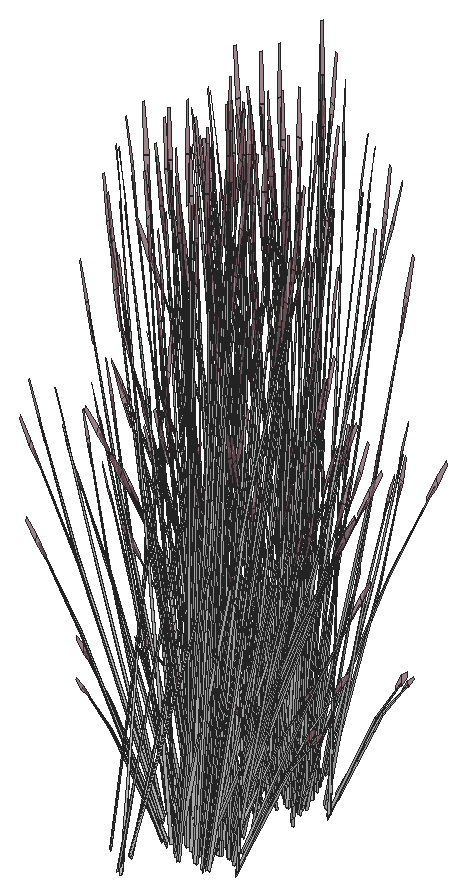
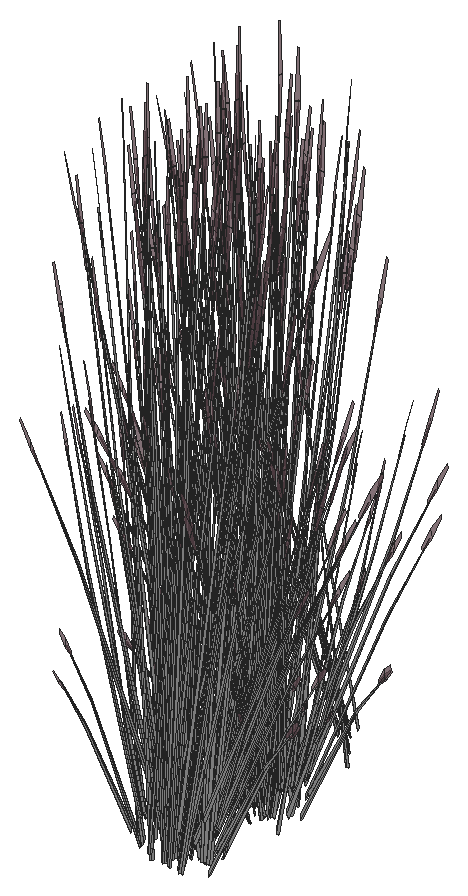
# SketchUp Ruby script. Lengths in inches.
U = 1.inch
M = Sketchup.active_model
def pt(a) = Geom::Point3d.new(a.map { |v| v * U })
def face(e, loops, mat)
  f = e.add_face(loops[0].map { |a| pt(a) })
  loops[1..].each { |l| e.add_face(l.map { |a| pt(a) }).erase! }
  f.material = f.back_material = mat if mat
  f
end
# faces: each face lists its corners as indices into pts; further lists are holes
def faces(e, pts, list, mat = nil) = list.each { |f| face(e, (f[0].is_a?(Array) ? f : [f]).map { |l| l.map { |i| pts[i] } }, mat) }
# xy, xz, yz: faces in a plane at the given z, y or x. An outline is a flat list of corners, or four numbers for a rectangle; further outlines are holes
def ring(l) = l.size == 4 ? [[l[0], l[1]], [l[2], l[1]], [l[2], l[3]], [l[0], l[3]]] : l.each_slice(2).to_a
def flat(e, list, mat, &to3) = list.each { |f| face(e, (f[0].is_a?(Array) ? f : [f]).map { |l| ring(l).map { |u, v| to3.(u, v) } }, mat) }
def xy(e, z, list, mat = nil) = flat(e, list, mat) { |x, y| [x, y, z] }
def xz(e, y, list, mat = nil) = flat(e, list, mat) { |x, z| [x, y, z] }
def yz(e, x, list, mat = nil) = flat(e, list, mat) { |y, z| [x, y, z] }
def lines(e, pts, list) = list.each { |a, b| e.add_line(pt(pts[a]), pt(pts[b])) }
# prism: a flat outline (further loops are holes) pulled along v
def prism(e, loops, v, mat = nil)
  f = face(e, loops, mat); d = Geom::Vector3d.new(v.map { |x| x * U })
  f.pushpull(f.normal.samedirection?(d) ? d.length : -d.length)
end
def box(e, o, s, mat = nil) = prism(e, [[o, [o[0] + s[0], o[1], o[2]], [o[0] + s[0], o[1] + s[1], o[2]], [o[0], o[1] + s[1], o[2]]]], [0, 0, s[2]], mat)
def at(x, y, z, deg = 0) = Geom::Transformation.translation(pt([x, y, z])) * Geom::Transformation.rotation(ORIGIN, Z_AXIS, deg.degrees)
def axes(o, x, y, z) = Geom::Transformation.new([*x, 0, *y, 0, *z, 0, *pt(o).to_a, 1])
def part(name) = M.definitions.add(name)
# library, detail: a bought-in or finely detailed component or shape, given as its bounding box
def library(name, o, s) = part(name).tap { |d| box(d.entities, o, s) }
def detail(e, o, s) = box(e.add_group.entities, o, s)
def put(e, d, t, mat = nil) = e.add_instance(d, t).tap { |i| i.material = mat if mat }
def group(e, t, mat = nil) = e.add_group.tap { |g| g.transformation = t; g.material = mat if mat }.entities
root = M.entities
M.materials.add("LightPink_Translucent").color = [144, 107, 117]
M.materials["LightPink_Translucent"].alpha = 0.75
M.materials.add("[_0053_Ivory_]").color = [200, 200, 200]
c1 = part("blade")
p = [[2.15,0.21,22],[0,0.17,0],[0.09,0.45,0],[2.18,0.31,22],[2.29,0.31,22],[0.38,0.45,0],
  [2.48,0.24,33],[2.49,0.24,33],[2.48,0.22,33]]
faces(c1.entities,p,[[0,1,2,3],[4,5,2,3],[6,3,4,7],[8,0,3,6]])
c2 = part("seeds")
p = [[0.3,-0.1,1.38],[-0.01,-0.03,1.59],[-0.01,-0.03,0.03],[0.14,-0.07,-0.07],[0.29,-0.03,3],[0.15,0.01,3.11]]
faces(c2.entities,p,[[0,1,2,3],[1,0,4,5]],"LightPink_Translucent")
c3 = part("blade with seeds")
put(c3.entities,c1,at(0,0,0))
put(c3.entities,c2,axes([2.4,0.25,30.99],[1.5799,-0.05474,1.17369],[-0.12525,1.92788,0.29478],[-0.07173,-0.02425,1.56792]))
put(root,c3,axes([679.4,325.39,38.18],[-0.1831,0.48359,-0.35414],[-0.53419,-0.14105,0.4572],[0.04898,0.1947,0.87481]),"[_0053_Ivory_]")
put(root,c3,axes([677.35,331.33,36.24],[0.11858,0.17508,1.43002],[-0.27325,0.4759,-0.30754],[-0.28057,-0.11375,0.61141]),"[_0053_Ivory_]")
put(root,c3,axes([679.41,330.5,35.68],[0.56663,0.1556,-0.30978],[-0.14267,0.54795,0.30978],[0.11423,-0.06319,1.38974]),"[_0053_Ivory_]")
put(root,c3,axes([678.25,324.45,38.99],[-0.0158,0.58168,-0.7886],[-0.66548,-0.03907,0.09517],[-0.07023,0.24643,1.11556]),"[_0053_Ivory_]")
put(root,c3,axes([677.83,331.17,38.63],[-0.60713,-0.01514,-0.71045],[0.04078,-0.63759,0.08574],[-0.25721,-0.06729,1.00501]),"[_0053_Ivory_]")
put(root,c3,axes([678.88,324.04,37.53],[-0.01487,-0.24136,1.71376],[0.64429,0.16012,0.13857],[-0.03985,0.34396,0.73262]),"[_0053_Ivory_]")
put(root,c3,axes([679.46,324.95,38.63],[0.28988,0.51132,-0.71045],[-0.59671,0.28496,0.08574],[0.06778,0.24706,1.00501]),"[_0053_Ivory_]")
put(root,c3,axes([677.8,332.4,35.98],[-0.56493,0.5287,0.30756],[-0.56528,-0.52313,-0.36492],[-0.01973,-0.15014,1.64885]),"[_0053_Ivory_]")
put(root,c3,axes([677.78,325.76,36.24],[0.19166,-0.0992,1.43002],[0.4732,0.29912,-0.30754],[-0.14084,0.25882,0.61141]),"[_0053_Ivory_]")
put(root,c3,axes([679.6,332.65,36.09],[0.68433,0.30479,0.24065],[-0.32934,0.63331,0.50002],[0,-0.14599,1.60543]),"[_0053_Ivory_]")
put(root,c3,axes([679.33,333.5,36.09],[0.16098,-0.74515,-0.23429],[0.76326,0.12989,0.51271],[-0.13337,-0.1029,1.5644]),"[_0053_Ivory_]")
put(root,c3,axes([677.63,331.3,38.33],[-0.44101,0.41656,-0.51099],[-0.38623,-0.44004,-0.3958],[-0.22407,-0.06338,0.97773]),"[_0053_Ivory_]")
put(root,c3,axes([676.64,331.86,36.42],[0.38775,-0.045,1.1486],[-0.24596,0.39648,0.84392],[-0.19161,-0.05948,0.25299]),"[_0053_Ivory_]")
put(root,c3,axes([679.38,332.22,36.37],[-0.65953,0.03882,0.44739],[-0.05964,-0.64439,-0.21531],[0.11807,-0.06531,1.43643]),"[_0053_Ivory_]")
put(root,c3,axes([677.68,332.69,36.13],[0,0.62885,0.49651],[-0.67951,0,0],[0,-0.14322,1.57504]),"[_0053_Ivory_]")
put(root,c3,axes([682.45,332.83,38.33],[0.16454,-0.57202,-0.51099],[0.56413,0.19607,-0.3958],[0.22713,-0.05245,0.97773]),"[_0053_Ivory_]")
put(root,c3,axes([678.03,325.27,37.02],[0.01334,-0.32463,1.54345],[0.60018,0.17147,0.21329],[-0.052,0.34598,0.72882]),"[_0053_Ivory_]")
put(root,c3,axes([681.55,330.5,36.03],[0.37973,-0.63014,0],[0.6353,0.35142,-0.51607],[0.14469,0.08004,1.63711]),"[_0053_Ivory_]")
put(root,c3,axes([677.08,331.75,37.53],[0.25192,-0.01424,1.71376],[-0.16712,0.61729,0.13857],[-0.35901,-0.03818,0.73262]),"[_0053_Ivory_]")
put(root,c3,axes([679.28,333.2,35.86],[-0.36485,-0.52782,-0.44739],[0.55265,-0.37168,0.21531],[-0.11807,-0.06531,1.43643]),"[_0053_Ivory_]")
put(root,c3,axes([679.36,332.45,36.01],[0.26406,0.70318,0.45755],[-0.7545,0.24452,0.17955],[0.00922,-0.12921,1.58856]),"[_0053_Ivory_]")
put(root,c3,axes([683.05,332.99,35.64],[-0.39118,0.07547,1.41583],[-0.06226,-0.6007,0.08104],[0.27398,-0.09092,0.80566]),"[_0053_Ivory_]")
put(root,c3,axes([683.76,332.46,35.91],[-0.37654,-0.40212,-0.06488],[0.4124,-0.36845,-0.29416],[0.11685,-0.02594,0.97024]),"[_0053_Ivory_]")
put(root,c3,axes([679.22,333.01,36.37],[-0.29468,0.56664,0.44739],[-0.61229,-0.27271,-0.21531],[0,-0.13062,1.43643]),"[_0053_Ivory_]")
put(root,c3,axes([680.31,332.51,35.86],[0,-0.72763,0],[0.75945,0,0],[0,0,1.79456]),"[_0053_Ivory_]")
put(root,c3,axes([681.23,330.83,36.13],[-0.56842,-0.31443,0.49651],[0.33976,-0.56381,0],[0.12946,0.07161,1.57504]),"[_0053_Ivory_]")
put(root,c3,axes([682.34,333.04,38.63],[0.53369,-0.27773,-0.71045],[0.29743,0.5717,0.08574],[0.25786,-0.06494,1.00501]),"[_0053_Ivory_]")
put(root,c3,axes([678.95,333.4,35.71],[-0.63179,-0.1031,-0.62353],[0.13332,-0.63596,-0.16365],[-0.18854,-0.07706,1.37633]),"[_0053_Ivory_]")
put(root,c3,axes([679.95,332.06,36.01],[-0.50358,0.57069,0.45755],[-0.59827,-0.50377,0.17955],[0.1214,-0.05695,1.58856]),"[_0053_Ivory_]")
put(root,c3,axes([680.5,333.08,35.95],[-0.56493,-0.54126,-0.06131],[0.56528,-0.54159,0],[-0.01973,-0.0189,1.75571]),"[_0053_Ivory_]")
put(root,c3,axes([679.07,331.12,36.13],[-0.17545,0.62497,0.17642],[-0.64204,-0.17686,0.35086],[0.11091,-0.00304,1.60407]),"[_0053_Ivory_]")
put(root,c3,axes([678.81,331.62,35.25],[-0.59782,0.25177,1.28929],[-0.19028,-0.72239,0.50096],[0.36709,0.01202,1.46642]),"[_0053_Ivory_]")
put(root,c3,axes([680.41,331.8125,36.27],[0.11717,-0.56122,0.1448],[0.57245,0.09742,-0.41347],[0.10418,0.05763,1.26744]),"[_0053_Ivory_]")
put(root,c3,axes([679.42,333.14,36.01],[0.76764,0.13249,0.45755],[-0.15622,0.74829,0.17955],[-0.11218,-0.07226,1.58856]),"[_0053_Ivory_]")
put(root,c3,axes([683.48,332.6,35.15],[-0.03174,-0.09547,1.76342],[0.22015,-0.55846,-0.26939],[0.22208,-0.00803,0.30037]),"[_0053_Ivory_]")
put(root,c3,axes([676.92,332.5,35.15],[0.0154,0.09911,1.76342],[-0.31051,0.51756,-0.26939],[-0.22056,-0.02609,0.30037]),"[_0053_Ivory_]")
put(root,c3,axes([680.17,331.96,36.37],[-0.36485,-0.52782,0.44739],[0.55265,-0.37168,-0.21531],[0.11807,0.06531,1.43643]),"[_0053_Ivory_]")
put(root,c3,axes([678.28,334.37,35.68],[-0.14267,-0.54795,-0.30978],[0.56663,-0.1556,0.30978],[-0.11423,-0.06319,1.38974]),"[_0053_Ivory_]")
put(root,c3,axes([679.01,334.34,36.13],[0.65264,-0.16691,0.17642],[0.16115,0.62115,0.35086],[-0.05821,-0.0905,1.60407]),"[_0053_Ivory_]")
put(root,c3,axes([680.35,331.99,36.32],[0.61322,-0.4175,-0.29095],[0.40778,0.58992,-0.50002],[0.1513,0.05991,1.59708]),"[_0053_Ivory_]")
put(root,c3,axes([682.79,333.09,38.18],[0.50475,0.17543,-0.35414],[-0.14722,0.5118,0.4572],[0.20322,-0.04693,0.87481]),"[_0053_Ivory_]")
put(root,c3,axes([678.125,334.61,35.67],[-0.56842,-0.31443,-0.49651],[0.33976,-0.56381,0],[-0.12946,-0.07161,1.57504]),"[_0053_Ivory_]")
put(root,c3,axes([681.9,330.88,35.67],[0.56842,0.31443,-0.49651],[-0.33976,0.56381,0],[0.12946,0.07161,1.57504]),"[_0053_Ivory_]")
put(root,c3,axes([676.86,332.28,38.18],[-0.50475,-0.17543,-0.35414],[0.14722,-0.5118,0.4572],[-0.20322,0.04693,0.87481]),"[_0053_Ivory_]")
put(root,c3,axes([680.82,332.68,35.86],[0.67951,0,0],[0,0.65103,0],[0,0,1.78407]),"[_0053_Ivory_]")
put(root,c3,axes([679.67,333.5,36.32],[-0.61322,0.4175,-0.29095],[-0.40778,-0.58992,-0.50002],[-0.1513,-0.05991,1.59708]),"[_0053_Ivory_]")
put(root,c3,axes([681.01,331.15,36.13],[-0.65264,0.16691,0.17642],[-0.16115,-0.62115,0.35086],[0.05821,0.0905,1.60407]),"[_0053_Ivory_]")
put(root,c3,axes([681.42,332.46,37.53],[-0.25192,0.01424,1.71376],[0.16712,-0.61729,0.13857],[0.35901,0.03818,0.73262]),"[_0053_Ivory_]")
put(root,c3,axes([681.74,331.12,35.68],[0.14267,0.54795,-0.30978],[-0.56663,0.1556,0.30978],[0.11423,0.06319,1.38974]),"[_0053_Ivory_]")
put(root,c3,axes([680.6,332.35,36.03],[-0.76764,-0.13249,0.49198],[0.15622,-0.74829,0.19306],[0.11218,0.07226,1.70813]),"[_0053_Ivory_]")
put(root,c3,axes([679.99,334.19,35.86],[-0.19817,-0.54216,0],[0.56587,-0.18986,0],[0,0,1.54371]),"[_0053_Ivory_]")
put(root,c3,axes([679.61,333.68,36.27],[-0.11717,0.56122,0.1448],[-0.57245,-0.09742,-0.41347],[-0.10418,-0.05763,1.26744]),"[_0053_Ivory_]")
put(root,c3,axes([680.73,334.12,35.84],[0.63764,-0.21337,-0.19198],[0.22406,0.61462,0.00008],[0.07038,-0.02358,1.73897]),"[_0053_Ivory_]")
put(root,c3,axes([680.95,334.375,36.13],[0.17545,-0.62497,0.17642],[0.64204,0.17686,0.35086],[-0.11091,0.00304,1.60407]),"[_0053_Ivory_]")
put(root,c3,axes([680.81,332.96,35.87],[0.42396,0.40619,0],[-0.42396,0.40619,0],[0,0,1.69266]),"[_0053_Ivory_]")
put(root,c3,axes([678.4,332.19,37],[0.17264,-0.09097,1.77064],[0.05953,0.63516,0.13857],[-0.37394,0.08428,0.63284]),"[_0053_Ivory_]")
put(root,c3,axes([681.95,332.78,36.13],[-0.47719,-0.45806,0.17642],[0.48088,-0.44429,0.35086],[-0.0527,0.09355,1.60407]),"[_0053_Ivory_]")
put(root,c3,axes([681.07,332.09,35.71],[0.63179,0.1031,-0.62353],[-0.13332,0.63596,-0.16365],[0.18854,0.07706,1.37633]),"[_0053_Ivory_]")
put(root,c3,axes([683.86,333.2,36.42],[-0.37526,0.10382,1.1486],[0.17664,-0.42906,0.84392],[0.19907,0.02936,0.25299]),"[_0053_Ivory_]")
put(root,c3,axes([679.85,334.4375,35.85],[-0.61229,-0.28233,0],[0.29468,-0.58663,0],[0,0,1.62707]),"[_0053_Ivory_]")
put(root,c3,axes([680.36,333.6875,36.12],[-0.59306,-0.50614,-0.25192],[0.49904,-0.56836,0.5513],[-0.1597,0.05921,1.68216]),"[_0053_Ivory_]")
put(root,c3,axes([678.8,334.66,36.13],[0.56842,0.31443,0.49651],[-0.33976,0.56381,0],[-0.12946,-0.07161,1.57504]),"[_0053_Ivory_]")
put(root,c3,axes([680.8,332.48,36.37],[0.29468,-0.56664,0.44739],[0.61229,0.27271,-0.21531],[0,0.13062,1.43643]),"[_0053_Ivory_]")
put(root,c3,axes([680.6875,332.8,35.95],[0,0.72727,-0.05637],[-0.75945,0,0],[0,0.02286,1.79368]),"[_0053_Ivory_]")
put(root,c3,axes([677.21,332.54,38.33],[-0.16454,0.57202,-0.51099],[-0.56413,-0.19607,-0.3958],[-0.22713,0.05245,0.97773]),"[_0053_Ivory_]")
put(root,c3,axes([680.74,332.29,35.86],[0.36485,0.52782,-0.44739],[-0.55265,0.37168,0.21531],[0.11807,0.06531,1.43643]),"[_0053_Ivory_]")
put(root,c3,axes([683.21,334.52,37.58],[-0.11624,-0.52862,-0.03492],[0.54943,-0.12153,-0.15832],[0.11473,0.03351,0.52218]),"[_0053_Ivory_]")
put(root,c3,axes([678.47,334.99,36.03],[-0.37973,0.63014,0],[-0.6353,-0.35142,-0.51607],[-0.14469,-0.08004,1.63711]),"[_0053_Ivory_]")
put(root,c3,axes([682.35,332.8,36.13],[0,-0.62885,0.49651],[0.67951,0,0],[0,0.14322,1.57504]),"[_0053_Ivory_]")
put(root,c3,axes([680.65,333.27,36.37],[0.65953,-0.03882,0.44739],[0.05964,0.64439,-0.21531],[-0.11807,0.06531,1.43643]),"[_0053_Ivory_]")
put(root,c3,axes([681.06,332.61,36.27],[0.56587,-0.18339,0.1448],[0.19817,0.52368,-0.41347],[0,0.11525,1.26744]),"[_0053_Ivory_]")
put(root,c3,axes([680.06,333.58,35.86],[-0.65953,0.03882,-0.44739],[-0.05964,-0.64439,0.21531],[-0.11807,0.06531,1.43643]),"[_0053_Ivory_]")
put(root,c3,axes([683.16,333.89,36.24],[-0.14627,-0.15466,1.43002],[0.19032,-0.51164,-0.30754],[0.29594,0.06931,0.61141]),"[_0053_Ivory_]")
put(root,c3,axes([680.55,334.45,35.86],[0.61229,0.28233,0],[-0.29468,0.58663,0],[0,0,1.74954]),"[_0053_Ivory_]")
put(root,c3,axes([680.79,335.07,35.85],[-0.37499,-0.63235,-0.05142],[0.6353,-0.35142,0.51607],[-0.15655,0.0602,1.6363]),"[_0053_Ivory_]")
put(root,c3,axes([680.66,333.54,36.27],[0.44871,0.37783,0.1448],[-0.37428,0.42627,-0.41347],[-0.10418,0.05763,1.26744]),"[_0053_Ivory_]")
put(root,c3,axes([677.1875,332.83,37.53],[0.21074,-0.13302,1.71376],[0.17741,0.61464,0.13857],[-0.33083,0.13891,0.73262]),"[_0053_Ivory_]")
put(root,c3,axes([678.49,340.97,37.53],[0.13883,0.2019,1.71376],[-0.64153,0.16998,0.13857],[-0.14499,-0.31697,0.73262]),"[_0053_Ivory_]")
put(root,c3,axes([681.82,334.2,38.63],[0.60713,0.01514,-0.71045],[-0.04078,0.63759,0.08574],[0.25721,0.06729,1.00501]),"[_0053_Ivory_]")
put(root,c3,axes([681.13,334.71,36.13],[0.56842,-0.31443,0.49651],[0.33976,0.56381,0],[-0.12946,0.07161,1.57504]),"[_0053_Ivory_]")
put(root,c3,axes([680.32,334.21,35.94],[0.26406,0.72244,-0.06012],[-0.7545,0.25315,0],[0.00922,0.02523,1.72173]),"[_0053_Ivory_]")
put(root,c3,axes([680.62,334.99,35.68],[-0.56663,-0.1556,-0.30978],[0.14267,-0.54795,0.30978],[-0.11423,0.06319,1.38974]),"[_0053_Ivory_]")
put(root,c3,axes([680.98,340.68,36.24],[-0.17264,0.12729,1.43002],[-0.51703,-0.22279,-0.30754],[0.09584,-0.27707,0.61141]),"[_0053_Ivory_]")
put(root,c3,axes([680.2,341.12,38.63],[-0.28988,-0.51132,-0.71045],[0.59671,-0.28496,0.08574],[-0.06778,-0.24706,1.00501]),"[_0053_Ivory_]")
put(root,c3,axes([676.53,333.88,36.24],[0.21107,0.05162,1.43002],[0.13604,0.52729,-0.30754],[-0.28671,0.0987,0.61141]),"[_0053_Ivory_]")
put(root,c3,axes([682.81,332.9,36.03],[0.75945,0,0],[0,0.70283,-0.51607],[0,0.16007,1.63711]),"[_0053_Ivory_]")
put(root,c3,axes([678.3125,340.4375,36.24],[-0.03678,0.20572,1.43002],[-0.53767,0.17221,-0.30754],[-0.12568,-0.26589,0.61141]),"[_0053_Ivory_]")
put(root,c3,axes([682.51,333.26,35.85],[-0.75908,-0.00503,-0.04976],[0,-0.70283,0.49943],[-0.02386,0.16,1.58352]),"[_0053_Ivory_]")
put(root,c3,axes([680.86,332.65,36.32],[0.68399,0.30005,-0.29095],[-0.32934,0.63331,-0.50002],[0.0215,0.15549,1.59708]),"[_0053_Ivory_]")
put(root,c3,axes([679.7,339.99,35.15],[-0.10187,0.02266,1.76342],[-0.56336,-0.25503,-0.26939],[0.00945,-0.21273,0.30037]),"[_0053_Ivory_]")
put(root,c3,axes([676.09,334.99,36.42],[0.25312,-0.28501,1.1486],[0.09988,0.45119,0.84392],[-0.18292,0.08079,0.25299]),"[_0053_Ivory_]")
put(root,c3,axes([682.18,334.46,38.18],[0.34557,0.39372,-0.35414],[-0.39459,0.37271,0.4572],[0.20048,0.05671,0.87481]),"[_0053_Ivory_]")
put(root,c3,axes([682.35,333.37,35.68],[-0.42396,0.39235,-0.30978],[-0.42396,-0.39235,0.30978],[0,0.12637,1.38974]),"[_0053_Ivory_]")
put(root,c3,axes([680.52,333.4,36.32],[0.07077,0.71755,-0.29095],[-0.73712,0.04339,-0.50002],[-0.1298,0.09558,1.59708]),"[_0053_Ivory_]")
put(root,c3,axes([680.79,333.125,35.86],[-0.29468,0.56664,-0.44739],[-0.61229,-0.27271,0.21531],[0,0.13062,1.43643]),"[_0053_Ivory_]")
put(root,c3,axes([677.04,333.75,38.18],[-0.52868,0.08987,-0.35414],[-0.1396,-0.51376,0.4572],[-0.1515,0.13799,0.87481]),"[_0053_Ivory_]")
put(root,c3,axes([681.4,341.62,38.63],[0.0158,-0.58168,-0.71045],[0.66548,0.03907,0.08574],[0.07023,-0.24643,1.00501]),"[_0053_Ivory_]")
put(root,c3,axes([680.25,340.6875,38.18],[0.1831,-0.48359,-0.35414],[0.53419,0.14105,0.4572],[-0.04898,-0.1947,0.87481]),"[_0053_Ivory_]")
put(root,c3,axes([680.65,341.33,37.53],[-0.11309,0.21615,1.71376],[-0.47441,-0.44731,0.13857],[0.21402,-0.27879,0.73262]),"[_0053_Ivory_]")
put(root,c3,axes([680.08,333.95,35.71],[-0.40909,0.47266,-0.62353],[-0.50819,-0.4286,-0.16365],[-0.16393,0.11791,1.37633]),"[_0053_Ivory_]")
put(root,c3,axes([679.98,341.02,38.33],[-0.59704,-0.15764,-0.51099],[0.20464,-0.54049,-0.3958],[-0.05475,-0.21761,0.97773]),"[_0053_Ivory_]")
put(root,c3,axes([680.35,339.67,36.42],[0.07791,0.3667,1.1486],[-0.43222,-0.2031,0.84392],[0.04651,-0.18776,0.25299]),"[_0053_Ivory_]")
put(root,c3,axes([680.81,334.75,35.98],[0.76036,0.2044,0.30756],[-0.19023,0.7306,-0.36492],[-0.12585,0.09144,1.64885]),"[_0053_Ivory_]")
put(root,c3,axes([681.27,341.43,38.33],[-0.43478,-0.42253,-0.51099],[0.45929,-0.37004,-0.3958],[0.06615,-0.21468,0.97773]),"[_0053_Ivory_]")
put(root,c3,axes([680.75,335.24,35.67],[-0.56842,0.31443,-0.49651],[-0.33976,-0.56381,0],[-0.12946,0.07161,1.57504]),"[_0053_Ivory_]")
put(root,c3,axes([682.64,333.38,35.67],[0,0.62885,-0.49651],[-0.67951,0,0],[0,0.14322,1.57504]),"[_0053_Ivory_]")
put(root,c3,axes([680.94,333.45,37.53],[-0.2256,-0.10835,1.71376],[0.46687,-0.45453,0.13857],[0.29098,0.20505,0.73262]),"[_0053_Ivory_]")
put(root,c3,axes([681.78,334.68,36.42],[-0.34197,-0.18082,1.1486],[0.44156,-0.18372,0.84392],[0.1191,0.15563,0.25299]),"[_0053_Ivory_]")
put(root,c3,axes([677.96,333.25,37.53],[0.1517,-0.19322,1.71376],[0.38303,0.52154,0.13857],[-0.26271,0.23751,0.73262]),"[_0053_Ivory_]")
put(root,c3,axes([681.68,341.27,38.18],[0.41095,-0.33109,-0.35414],[0.38901,0.37805,0.4572],[0.05919,-0.19208,0.87481]),"[_0053_Ivory_]")
put(root,c3,axes([678.125,340.11,36.42],[0.31682,0.21887,1.1486],[-0.4614,0.13157,0.84392],[-0.09872,-0.16821,0.25299]),"[_0053_Ivory_]")
put(root,c3,axes([678.89,341.27,38.63],[-0.51789,-0.30395,-0.71045],[0.36805,-0.53263,0.08574],[-0.18764,-0.18149,1.00501]),"[_0053_Ivory_]")
put(root,c3,axes([677.48,333.8125,38.33],[0.15602,0.5742,-0.51099],[-0.59087,0.10045,-0.3958],[-0.16933,0.15423,0.97773]),"[_0053_Ivory_]")
put(root,c3,axes([678.71,340.86,38.18],[-0.0938,-0.50652,-0.35414],[0.53623,-0.13375,0.4572],[-0.14403,-0.14515,0.87481]),"[_0053_Ivory_]")
put(root,c3,axes([681.27,335.14,36.03],[0.37973,0.63014,0],[-0.6353,0.35142,-0.51607],[-0.14469,0.08004,1.63711]),"[_0053_Ivory_]")
put(root,c3,axes([681.87,335.36,35.15],[0.04425,-0.09079,1.76342],[0.55709,-0.26738,-0.26939],[0.16889,0.13839,0.30037]),"[_0053_Ivory_]")
put(root,c3,axes([680.94,332.65,36.5],[-0.01659,-0.59209,1.41272],[0.75089,0.15348,0.59816],[-0.1776,0.32398,1.3335]),"[_0053_Ivory_]")
put(root,c3,axes([681.14,333.29,35.75],[0.2227,0.57576,-0.69212],[-0.64151,0.20736,-0.18165],[0.02462,0.19497,1.52773]),"[_0053_Ivory_]")
put(root,c3,axes([676.76,335.28,35.15],[0.08147,0.06283,1.76342],[0.13814,0.58211,-0.26939],[-0.18056,0.12413,0.30037]),"[_0053_Ivory_]")
put(root,c3,axes([681,334.93,38.33],[0.59932,-0.14948,-0.51099],[0.10484,0.56611,-0.3958],[0.16097,0.16223,0.97773]),"[_0053_Ivory_]")
put(root,c3,axes([677.875,340.77,35.15],[-0.05883,0.08284,1.76342],[-0.59454,0.17861,-0.26939],[-0.14363,-0.16248,0.30037]),"[_0053_Ivory_]")
put(root,c3,axes([681.83,335.51,36.32],[-0.38947,-0.01972,1.0506],[0.25721,-0.41888,0.58006],[0.15386,0.14882,0.8241]),"[_0053_Ivory_]")
put(root,c3,axes([678.86,343.04,35.75],[-0.24943,-0.64486,-0.69835],[0.71849,-0.23224,-0.18329],[-0.02757,-0.21836,1.54149]),"[_0053_Ivory_]")
put(root,c3,axes([677.56,341.6,37.53],[0.2256,0.10835,1.71376],[-0.46687,0.45453,0.13857],[-0.29098,-0.20505,0.73262]),"[_0053_Ivory_]")
put(root,c3,axes([682.19,341.07,35.15],[-0.0909,-0.04954,1.76342],[-0.2335,-0.55347,-0.26939],[0.15752,-0.1502,0.30037]),"[_0053_Ivory_]")
put(root,c3,axes([678.65,341.28,38.33],[-0.59932,0.14948,-0.51099],[-0.10484,-0.56611,-0.3958],[-0.16097,-0.16223,0.97773]),"[_0053_Ivory_]")
put(root,c3,axes([677.84,333.72,37.53],[0.11309,-0.21615,1.71376],[0.47441,0.44731,0.13857],[-0.21402,0.27879,0.73262]),"[_0053_Ivory_]")
put(root,c3,axes([680.56,334.49,36.24],[0.01072,-0.20846,1.43002],[0.51218,-0.23285,-0.30754],[0.15811,0.2495,0.61141]),"[_0053_Ivory_]")
put(root,c3,axes([682.1875,342.63,38.63],[0.31725,-0.49618,-0.71045],[0.55593,0.35263,0.08574],[0.18942,-0.17977,1.00501]),"[_0053_Ivory_]")
put(root,c3,axes([678.76,341.1875,36.03],[-0.37973,-0.63014,0],[0.6353,-0.35142,-0.51607],[0.14469,-0.08004,1.63711]),"[_0053_Ivory_]")
put(root,c3,axes([682.17,342.4,38.33],[-0.15602,-0.5742,-0.51099],[0.59087,-0.10045,-0.3958],[0.16933,-0.15423,0.97773]),"[_0053_Ivory_]")
put(root,c3,axes([677.97,334.94,38.18],[-0.41095,0.33109,-0.35414],[-0.38901,-0.37805,0.4572],[-0.05919,0.19208,0.87481]),"[_0053_Ivory_]")
put(root,c3,axes([679.59,340.43,35.78],[-0.4197,0.36076,-0.03893],[-0.38456,-0.39511,-0.17649],[-0.02707,-0.11196,0.58215]),"[_0053_Ivory_]")
put(root,c3,axes([678.24,336.23,36.42],[-0.01572,-0.37392,1.1486],[0.39276,0.26669,0.84392],[-0.07724,0.17822,0.25299]),"[_0053_Ivory_]")
put(root,c3,axes([679.27,335.34,35.15],[0.09829,-0.03422,1.76342],[0.59126,0.18834,-0.26939],[0.01729,0.21228,0.30037]),"[_0053_Ivory_]")
put(root,c3,axes([680.13,344.71,36.98],[0.52485,0.25358,1.51261],[-0.51417,0.54629,0.59816],[-0.23031,-0.32378,1.26806]),"[_0053_Ivory_]")
put(root,c3,axes([678.38,334.79,38.66],[0.43478,0.42253,-0.5672],[-0.45929,0.37004,-0.43934],[-0.06615,0.21468,1.08528]),"[_0053_Ivory_]")
put(root,c3,axes([677.39,342.95,35.67],[0,-0.62885,-0.49651],[0.67951,0,0],[0,-0.14322,1.57504]),"[_0053_Ivory_]")
put(root,c3,axes([679.27,341.09,35.67],[0.56842,-0.31443,-0.49651],[0.33976,0.56381,0],[0.12946,-0.07161,1.57504]),"[_0053_Ivory_]")
put(root,c3,axes([677.91,335.42,36.48],[0.55175,-0.11136,0.06507],[0.12684,0.44864,-0.86304],[-0.03498,0.22711,0.7736]),"[_0053_Ivory_]")
put(root,c3,axes([679.67,335.2,38.33],[0.59704,0.15764,-0.51099],[-0.20464,0.54049,-0.3958],[0.05475,0.21761,0.97773]),"[_0053_Ivory_]")
put(root,c3,axes([682.65,342.18,36.24],[-0.21697,-0.01863,1.43002],[-0.22228,-0.49966,-0.30754],[0.26655,-0.14135,0.61141]),"[_0053_Ivory_]")
put(root,c3,axes([680.01,334.08,37.53],[-0.13883,-0.2019,1.71376],[0.64153,-0.16998,0.13857],[0.14499,0.31697,0.73262]),"[_0053_Ivory_]")
put(root,c3,axes([679.95,342.38,35.71],[0.40909,-0.47266,-0.62353],[0.50819,0.4286,-0.16365],[0.16393,-0.11791,1.37633]),"[_0053_Ivory_]")
put(root,c3,axes([682.9,341.26,36.42],[-0.2023,0.32011,1.1486],[-0.17388,-0.43009,0.84392],[0.16708,-0.10777,0.25299]),"[_0053_Ivory_]")
put(root,c3,axes([679.4,335.53,38.18],[-0.1831,0.48359,-0.35414],[-0.53419,-0.14105,0.4572],[0.04898,0.1947,0.87481]),"[_0053_Ivory_]")
put(root,c3,axes([678.25,334.59,38.99],[-0.0158,0.58168,-0.7886],[-0.66548,-0.03907,0.09517],[-0.07023,0.24643,1.11556]),"[_0053_Ivory_]")
put(root,c3,axes([682.61,342.46,38.18],[0.52868,-0.08987,-0.35414],[0.1396,0.51376,0.4572],[0.1515,-0.13799,0.87481]),"[_0053_Ivory_]")
put(root,c3,axes([679.24,343.21,35.86],[0.29468,-0.56664,-0.44739],[0.61229,0.27271,0.21531],[0,-0.13062,1.43643]),"[_0053_Ivory_]")
put(root,c3,axes([677.47,341.76,38.18],[-0.34557,-0.39372,-0.35414],[0.39459,-0.37271,0.4572],[-0.20048,-0.05671,0.87481]),"[_0053_Ivory_]")
put(root,c3,axes([678.88,334.18,37.53],[-0.01487,-0.24136,1.71376],[0.64429,0.16012,0.13857],[-0.03985,0.34396,0.73262]),"[_0053_Ivory_]")
put(root,c3,axes([679.5,342.93,36.32],[-0.07077,-0.71755,-0.29095],[0.73712,-0.04339,-0.50002],[0.1298,-0.09558,1.59708]),"[_0053_Ivory_]")
put(root,c3,axes([677.68,342.97,35.68],[0.42396,-0.39235,-0.30978],[0.42396,0.39235,0.30978],[0,-0.12637,1.38974]),"[_0053_Ivory_]")
put(root,c3,axes([677.51,341.09,35.78],[-0.1752,0.51349,-0.03893],[-0.53924,-0.15795,-0.17649],[-0.08187,-0.08399,0.58215]),"[_0053_Ivory_]")
put(root,c3,axes([679.16,343.68,36.32],[-0.68399,-0.30005,-0.29095],[0.32934,-0.63331,-0.50002],[-0.0215,-0.15549,1.59708]),"[_0053_Ivory_]")
put(root,c3,axes([679.46,335.09,38.63],[0.28988,0.51132,-0.71045],[-0.59671,0.28496,0.08574],[0.06778,0.24706,1.00501]),"[_0053_Ivory_]")
put(root,c3,axes([677.22,343.43,36.03],[-0.75945,0,0],[0,-0.70283,-0.51607],[0,-0.16007,1.63711]),"[_0053_Ivory_]")
put(root,c3,axes([677.35,342.17,36.24],[0.11858,0.17508,1.43002],[-0.27325,0.4759,-0.30754],[-0.28057,-0.11375,0.61141]),"[_0053_Ivory_]")
put(root,c3,axes([677.78,335.9,36.24],[0.19166,-0.0992,1.43002],[0.4732,0.29912,-0.30754],[-0.14084,0.25882,0.61141]),"[_0053_Ivory_]")
put(root,c3,axes([679.41,341.34,35.68],[0.56663,0.1556,-0.30978],[-0.14267,0.54795,0.30978],[0.11423,-0.06319,1.38974]),"[_0053_Ivory_]")
put(root,c3,axes([677.83,342.02,38.63],[-0.60713,-0.01514,-0.71045],[0.04078,-0.63759,0.08574],[-0.25721,-0.06729,1.00501]),"[_0053_Ivory_]")
put(root,c3,axes([677.8,343.24,35.98],[-0.56493,0.5287,0.30756],[-0.56528,-0.52313,-0.36492],[-0.01973,-0.15014,1.64885]),"[_0053_Ivory_]")
put(root,c3,axes([678.03,335.41,37.02],[0.01334,-0.32463,1.54345],[0.60018,0.17147,0.21329],[-0.052,0.34598,0.72882]),"[_0053_Ivory_]")
put(root,c3,axes([679.6,343.49,36.09],[0.68433,0.30479,0.24065],[-0.32934,0.63331,0.50002],[0,-0.14599,1.60543]),"[_0053_Ivory_]")
put(root,c3,axes([679.33,344.35,36.09],[0.16098,-0.74515,-0.23429],[0.76326,0.12989,0.51271],[-0.13337,-0.1029,1.5644]),"[_0053_Ivory_]")
put(root,c3,axes([677.63,342.15,38.33],[-0.44101,0.41656,-0.51099],[-0.38623,-0.44004,-0.3958],[-0.22407,-0.06338,0.97773]),"[_0053_Ivory_]")
put(root,c3,axes([676.64,342.7,36.42],[0.38775,-0.045,1.1486],[-0.24596,0.39648,0.84392],[-0.19161,-0.05948,0.25299]),"[_0053_Ivory_]")
put(root,c3,axes([679.38,343.07,36.37],[-0.65953,0.03882,0.44739],[-0.05964,-0.64439,-0.21531],[0.11807,-0.06531,1.43643]),"[_0053_Ivory_]")
put(root,c3,axes([677.68,343.54,36.13],[0,0.62885,0.49651],[-0.67951,0,0],[0,-0.14322,1.57504]),"[_0053_Ivory_]")
put(root,c3,axes([682.45,343.68,38.33],[0.16454,-0.57202,-0.51099],[0.56413,0.19607,-0.3958],[0.22713,-0.05245,0.97773]),"[_0053_Ivory_]")
put(root,c3,axes([681.55,341.35,36.03],[0.37973,-0.63014,0],[0.6353,0.35142,-0.51607],[0.14469,0.08004,1.63711]),"[_0053_Ivory_]")
put(root,c3,axes([677.08,342.59,37.53],[0.25192,-0.01424,1.71376],[-0.16712,0.61729,0.13857],[-0.35901,-0.03818,0.73262]),"[_0053_Ivory_]")
put(root,c3,axes([679.28,344.04,35.86],[-0.36485,-0.52782,-0.44739],[0.55265,-0.37168,0.21531],[-0.11807,-0.06531,1.43643]),"[_0053_Ivory_]")
put(root,c3,axes([679.36,343.3,36.01],[0.26406,0.70318,0.45755],[-0.7545,0.24452,0.17955],[0.00922,-0.12921,1.58856]),"[_0053_Ivory_]")
put(root,c3,axes([683.05,343.84,35.64],[-0.39118,0.07547,1.41583],[-0.06226,-0.6007,0.08104],[0.27398,-0.09092,0.80566]),"[_0053_Ivory_]")
put(root,c3,axes([683.76,343.31,35.91],[-0.37654,-0.40212,-0.06488],[0.4124,-0.36845,-0.29416],[0.11685,-0.02594,0.97024]),"[_0053_Ivory_]")
put(root,c3,axes([679.22,343.85,36.37],[-0.29468,0.56664,0.44739],[-0.61229,-0.27271,-0.21531],[0,-0.13062,1.43643]),"[_0053_Ivory_]")
put(root,c3,axes([680.31,343.36,35.86],[0,-0.72763,0],[0.75945,0,0],[0,0,1.79456]),"[_0053_Ivory_]")
put(root,c3,axes([681.23,341.68,36.13],[-0.56842,-0.31443,0.49651],[0.33976,-0.56381,0],[0.12946,0.07161,1.57504]),"[_0053_Ivory_]")
put(root,c3,axes([682.34,343.88,38.63],[0.53369,-0.27773,-0.71045],[0.29743,0.5717,0.08574],[0.25786,-0.06494,1.00501]),"[_0053_Ivory_]")
put(root,c3,axes([678.95,344.25,35.71],[-0.63179,-0.1031,-0.62353],[0.13332,-0.63596,-0.16365],[-0.18854,-0.07706,1.37633]),"[_0053_Ivory_]")
put(root,c3,axes([679.95,342.9,36.01],[-0.50358,0.57069,0.45755],[-0.59827,-0.50377,0.17955],[0.1214,-0.05695,1.58856]),"[_0053_Ivory_]")
put(root,c3,axes([680.5,343.92,35.95],[-0.56493,-0.54126,-0.06131],[0.56528,-0.54159,0],[-0.01973,-0.0189,1.75571]),"[_0053_Ivory_]")
put(root,c3,axes([679.07,341.96,36.13],[-0.17545,0.62497,0.17642],[-0.64204,-0.17686,0.35086],[0.11091,-0.00304,1.60407]),"[_0053_Ivory_]")
put(root,c3,axes([678.81,342.46,35.25],[-0.59782,0.25177,1.28929],[-0.19028,-0.72239,0.50096],[0.36709,0.01202,1.46642]),"[_0053_Ivory_]")
put(root,c3,axes([680.41,342.65,36.27],[0.11717,-0.56122,0.1448],[0.57245,0.09742,-0.41347],[0.10418,0.05763,1.26744]),"[_0053_Ivory_]")
put(root,c3,axes([679.42,343.99,36.01],[0.76764,0.13249,0.45755],[-0.15622,0.74829,0.17955],[-0.11218,-0.07226,1.58856]),"[_0053_Ivory_]")
put(root,c3,axes([683.48,343.44,35.15],[-0.03174,-0.09547,1.76342],[0.22015,-0.55846,-0.26939],[0.22208,-0.00803,0.30037]),"[_0053_Ivory_]")
put(root,c3,axes([676.92,343.35,35.15],[0.0154,0.09911,1.76342],[-0.31051,0.51756,-0.26939],[-0.22056,-0.02609,0.30037]),"[_0053_Ivory_]")
put(root,c3,axes([680.17,342.8,36.37],[-0.36485,-0.52782,0.44739],[0.55265,-0.37168,-0.21531],[0.11807,0.06531,1.43643]),"[_0053_Ivory_]")
put(root,c3,axes([678.28,345.21,35.68],[-0.14267,-0.54795,-0.30978],[0.56663,-0.1556,0.30978],[-0.11423,-0.06319,1.38974]),"[_0053_Ivory_]")
put(root,c3,axes([679.01,345.18,36.13],[0.65264,-0.16691,0.17642],[0.16115,0.62115,0.35086],[-0.05821,-0.0905,1.60407]),"[_0053_Ivory_]")
put(root,c3,axes([680.35,342.84,36.32],[0.61322,-0.4175,-0.29095],[0.40778,0.58992,-0.50002],[0.1513,0.05991,1.59708]),"[_0053_Ivory_]")
put(root,c3,axes([682.79,343.9375,38.18],[0.50475,0.17543,-0.35414],[-0.14722,0.5118,0.4572],[0.20322,-0.04693,0.87481]),"[_0053_Ivory_]")
put(root,c3,axes([678.125,345.45,35.67],[-0.56842,-0.31443,-0.49651],[0.33976,-0.56381,0],[-0.12946,-0.07161,1.57504]),"[_0053_Ivory_]")
put(root,c3,axes([681.9,341.73,35.67],[0.56842,0.31443,-0.49651],[-0.33976,0.56381,0],[0.12946,0.07161,1.57504]),"[_0053_Ivory_]")
put(root,c3,axes([676.86,343.12,38.18],[-0.50475,-0.17543,-0.35414],[0.14722,-0.5118,0.4572],[-0.20322,0.04693,0.87481]),"[_0053_Ivory_]")
put(root,c3,axes([680.82,343.52,35.86],[0.67951,0,0],[0,0.65103,0],[0,0,1.78407]),"[_0053_Ivory_]")
put(root,c3,axes([679.67,344.34,36.32],[-0.61322,0.4175,-0.29095],[-0.40778,-0.58992,-0.50002],[-0.1513,-0.05991,1.59708]),"[_0053_Ivory_]")
put(root,c3,axes([681.01,341.99,36.13],[-0.65264,0.16691,0.17642],[-0.16115,-0.62115,0.35086],[0.05821,0.0905,1.60407]),"[_0053_Ivory_]")
put(root,c3,axes([681.42,343.3,37.53],[-0.25192,0.01424,1.71376],[0.16712,-0.61729,0.13857],[0.35901,0.03818,0.73262]),"[_0053_Ivory_]")
put(root,c3,axes([681.74,341.96,35.68],[0.14267,0.54795,-0.30978],[-0.56663,0.1556,0.30978],[0.11423,0.06319,1.38974]),"[_0053_Ivory_]")
put(root,c3,axes([680.6,343.1875,36.03],[-0.76764,-0.13249,0.49198],[0.15622,-0.74829,0.19306],[0.11218,0.07226,1.70813]),"[_0053_Ivory_]")
put(root,c3,axes([679.99,345.04,35.86],[-0.19817,-0.54216,0],[0.56587,-0.18986,0],[0,0,1.54371]),"[_0053_Ivory_]")
put(root,c3,axes([679.61,344.52,36.27],[-0.11717,0.56122,0.1448],[-0.57245,-0.09742,-0.41347],[-0.10418,-0.05763,1.26744]),"[_0053_Ivory_]")
put(root,c3,axes([680.73,344.96,35.84],[0.63764,-0.21337,-0.19198],[0.22406,0.61462,0.00008],[0.07038,-0.02358,1.73897]),"[_0053_Ivory_]")
put(root,c3,axes([680.95,345.22,36.13],[0.17545,-0.62497,0.17642],[0.64204,0.17686,0.35086],[-0.11091,0.00304,1.60407]),"[_0053_Ivory_]")
put(root,c3,axes([680.81,343.8,35.87],[0.42396,0.40619,0],[-0.42396,0.40619,0],[0,0,1.69266]),"[_0053_Ivory_]")
put(root,c3,axes([678.4,343.04,37],[0.17264,-0.09097,1.77064],[0.05953,0.63516,0.13857],[-0.37394,0.08428,0.63284]),"[_0053_Ivory_]")
put(root,c3,axes([681.95,343.62,36.13],[-0.47719,-0.45806,0.17642],[0.48088,-0.44429,0.35086],[-0.0527,0.09355,1.60407]),"[_0053_Ivory_]")
put(root,c3,axes([681.07,342.93,35.71],[0.63179,0.1031,-0.62353],[-0.13332,0.63596,-0.16365],[0.18854,0.07706,1.37633]),"[_0053_Ivory_]")
put(root,c3,axes([683.86,344.04,36.42],[-0.37526,0.10382,1.1486],[0.17664,-0.42906,0.84392],[0.19907,0.02936,0.25299]),"[_0053_Ivory_]")
put(root,c3,axes([679.85,345.28,35.85],[-0.61229,-0.28233,0],[0.29468,-0.58663,0],[0,0,1.62707]),"[_0053_Ivory_]")
put(root,c3,axes([680.36,344.53,36.12],[-0.59306,-0.50614,-0.25192],[0.49904,-0.56836,0.5513],[-0.1597,0.05921,1.68216]),"[_0053_Ivory_]")
put(root,c3,axes([678.8,345.5,36.13],[0.56842,0.31443,0.49651],[-0.33976,0.56381,0],[-0.12946,-0.07161,1.57504]),"[_0053_Ivory_]")
put(root,c3,axes([680.8,343.32,36.37],[0.29468,-0.56664,0.44739],[0.61229,0.27271,-0.21531],[0,0.13062,1.43643]),"[_0053_Ivory_]")
put(root,c3,axes([680.6875,343.65,35.95],[0,0.72727,-0.05637],[-0.75945,0,0],[0,0.02286,1.79368]),"[_0053_Ivory_]")
